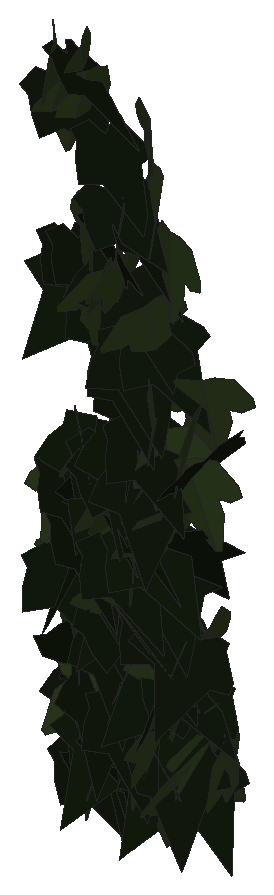
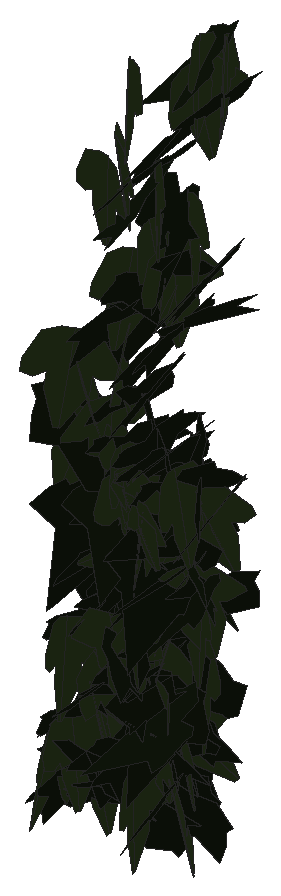
# SketchUp Ruby script. Lengths in inches.
U = 1.inch
M = Sketchup.active_model
def pt(a) = Geom::Point3d.new(a.map { |v| v * U })
def face(e, loops, mat)
  f = e.add_face(loops[0].map { |a| pt(a) })
  loops[1..].each { |l| e.add_face(l.map { |a| pt(a) }).erase! }
  f.material = f.back_material = mat if mat
  f
end
# faces: each face lists its corners as indices into pts; further lists are holes
def faces(e, pts, list, mat = nil) = list.each { |f| face(e, (f[0].is_a?(Array) ? f : [f]).map { |l| l.map { |i| pts[i] } }, mat) }
# xy, xz, yz: faces in a plane at the given z, y or x. An outline is a flat list of corners, or four numbers for a rectangle; further outlines are holes
def ring(l) = l.size == 4 ? [[l[0], l[1]], [l[2], l[1]], [l[2], l[3]], [l[0], l[3]]] : l.each_slice(2).to_a
def flat(e, list, mat, &to3) = list.each { |f| face(e, (f[0].is_a?(Array) ? f : [f]).map { |l| ring(l).map { |u, v| to3.(u, v) } }, mat) }
def xy(e, z, list, mat = nil) = flat(e, list, mat) { |x, y| [x, y, z] }
def xz(e, y, list, mat = nil) = flat(e, list, mat) { |x, z| [x, y, z] }
def yz(e, x, list, mat = nil) = flat(e, list, mat) { |y, z| [x, y, z] }
def lines(e, pts, list) = list.each { |a, b| e.add_line(pt(pts[a]), pt(pts[b])) }
# prism: a flat outline (further loops are holes) pulled along v
def prism(e, loops, v, mat = nil)
  f = face(e, loops, mat); d = Geom::Vector3d.new(v.map { |x| x * U })
  f.pushpull(f.normal.samedirection?(d) ? d.length : -d.length)
end
def box(e, o, s, mat = nil) = prism(e, [[o, [o[0] + s[0], o[1], o[2]], [o[0] + s[0], o[1] + s[1], o[2]], [o[0], o[1] + s[1], o[2]]]], [0, 0, s[2]], mat)
def at(x, y, z, deg = 0) = Geom::Transformation.translation(pt([x, y, z])) * Geom::Transformation.rotation(ORIGIN, Z_AXIS, deg.degrees)
def axes(o, x, y, z) = Geom::Transformation.new([*x, 0, *y, 0, *z, 0, *pt(o).to_a, 1])
def part(name) = M.definitions.add(name)
# library, detail: a bought-in or finely detailed component or shape, given as its bounding box
def library(name, o, s) = part(name).tap { |d| box(d.entities, o, s) }
def detail(e, o, s) = box(e.add_group.entities, o, s)
def put(e, d, t, mat = nil) = e.add_instance(d, t).tap { |i| i.material = mat if mat }
def group(e, t, mat = nil) = e.add_group.tap { |g| g.transformation = t; g.material = mat if mat }.entities
root = M.entities
M.materials.add("efeu1").color = [18, 25, 13]
M.materials.add("efeu2").color = [43, 57, 29]
c1 = part("ivyleaf_10")
p = [[0,0.5,-0.03],[-0.0625,2.02,-0.43],[-0.19,2.01,-0.46],[-0.54,1.05,-0.29],[-0.52,0.625,-0.18],[-0.83,0.76,-0.28],
  [-1.16,0.64,-0.33],[-1.15,0.33,-0.24],[-0.77,-0.39,0.02],[-0.3,-0.51,0.16],[0.04,-0.48,0.23],[-0.02,2.01,-0.4375],
  [-0.06,2.01,-0.43],[0.04,-0.49,0.23],[0.67,-0.49,0.14],[1.38,0.36,-0.2],[1.375,0.51,-0.24],[0.81,0.65,-0.19],
  [0.62,0.59,-0.15],[0.6,1.09,-0.28],[0.5,1.23,-0.31]]
faces(c1.entities,p,[[0,1,2,3,4,5,6,7,8,9,10],[11,12,0,13,14,15,16,17,18,19,20]],"efeu2")
c2 = part("ivyleaf_9")
p = [[1.54,2.16,1.25],[1.36,2.04,1.19],[-0.21,0.99,0.68],[-0.71,1.11,0.82],[-0.85,0.86,0.67],[-0.8,0.17,0.21],
  [-0.9,-0.01,0.1],[-0.67,-0.16,-0.02],[-0.08,-0.08,-0.05],[-0.03,-0.6,-0.4],[0.65,-0.88,-0.66],[0.83,-0.6,-0.49],
  [1.29,-0.42,-0.43],[1.8125,-0.07,-0.26],[1.21,0.44,0.15]]
faces(c2.entities,p,[[0,1,2,3,4,5,6,7,8,9,10,11,12,13,14]],"efeu1")
put(root,c1,axes([16.36,223.625,233.52],[0.23631,-0.40338,-0.17731],[0.01885,0.21027,-0.45324],[0.44023,0.20753,0.11459]))
put(root,c1,axes([16.68,224.23,224.14],[-0.34276,-0.05876,0.35925],[-0.26013,-0.30565,-0.29818],[0.25465,-0.39131,0.17896]))
put(root,c1,axes([16.51,223.875,224.82],[0.3091,-0.25368,-0.30017],[-0.09702,0.32081,-0.37103],[0.38084,0.28762,0.1491]))
put(root,c1,axes([16.57,224.01,225.79],[-0.41513,0.23915,0.1431],[-0.16261,0.00065,-0.47282],[-0.22633,-0.4391,0.07724]))
put(root,c1,axes([16.5,223.97,227.23],[0.42817,0.18988,-0.17497],[-0.17477,-0.03628,-0.46705],[-0.19007,0.46112,0.0353]))
put(root,c1,axes([16.59,224.15,226.13],[-0.37301,-0.2749,0.18786],[-0.09895,-0.17783,-0.45671],[0.31791,-0.3779,0.07826]))
put(root,c1,axes([16.54,224.35,227.62],[0.01144,-0.49941,-0.02146],[0.0006,0.02148,-0.49954],[0.49987,0.0114,0.0011]))
put(root,c1,axes([16.54,224.35,224.21],[0.31577,-0.36915,-0.1184],[-0.05573,0.1079,-0.48503],[0.38365,0.31951,0.027]))
put(root,c2,axes([16.54,224.18,229.95],[-0.30358,-0.34379,0.19911],[-0.01218,-0.24241,-0.43714],[0.3971,-0.27026,0.13881]))
put(root,c2,axes([16.3,223.8125,233.03],[0.23243,-0.37753,-0.23119],[-0.00634,0.25825,-0.4281],[0.44265,0.20194,0.11526]))
put(root,c2,axes([16.32,223.96,227.17],[0.2145,-0.44997,-0.03894],[-0.0152,0.03589,-0.49848],[0.45139,0.21504,0.00172]))
put(root,c2,axes([16.6,224.04,226.47],[-0.36619,0.11606,-0.32005],[0.28886,-0.14284,-0.3823],[-0.18017,-0.46489,0.03757]))
put(root,c2,axes([16.42,223.88,226.05],[-0.01712,-0.3956,-0.3053],[0.01443,0.30496,-0.39597],[0.4995,-0.02237,0.00097]))
put(root,c2,axes([16.35,224,230.5625],[0.21139,-0.4458,-0.0811],[-0.01887,0.08076,-0.49307],[0.45272,0.21153,0.01732]))
put(root,c2,axes([16.29,224.72,224.5625],[0.46602,-0.17972,-0.023],[0.04122,0.16698,-0.46949],[0.17644,0.43568,0.17044]))
put(root,c2,axes([16.45,223.98,226.22],[0.44251,-0.14345,-0.18333],[-0.1495,0.1267,-0.46],[0.17843,0.46192,0.06924]))
put(root,c1,axes([16.5625,224.32,224.05],[0.03575,0.4985,-0.01489],[-0.00064,-0.01489,-0.49978],[-0.49872,0.03575,-0.00042]))
put(root,c2,axes([16.62,224.4,224.64],[0.40758,0.24782,-0.14987],[-0.18534,0.02437,-0.46374],[-0.22254,0.43358,0.11173]))
put(root,c2,axes([16.39,224.16,230.51],[0.22114,-0.44173,-0.07729],[0.00508,0.08865,-0.49205],[0.44841,0.21684,0.0437]))
put(root,c2,axes([16.25,224.125,224.36],[0.16586,-0.02978,0.47075],[0.47156,-0.00133,-0.16623],[0.01115,0.49911,0.02765]))
put(root,c1,axes([16.66,223.76,233.48],[0.1131,-0.45719,-0.1679],[0.01562,0.17568,-0.46786],[0.48679,0.10059,0.05402]))
put(root,c1,axes([16.7,223.8,233.09],[-0.10581,-0.48456,0.06328],[0.00095,-0.06495,-0.49576],[0.48867,-0.1048,0.01467]))
put(root,c2,axes([16.9,223.6,227.79],[0.05176,0.11866,-0.48295],[-0.48804,0.10546,-0.0264],[0.0956,0.47413,0.12674]))
put(root,c2,axes([16.65,224.27,224.17],[-0.41082,-0.20004,-0.20299],[0.17385,0.1063,-0.45659],[0.22583,-0.44574,-0.01778]))
put(root,c1,axes([16.66,224.55,224.54],[-0.36664,0.32625,-0.09557],[-0.00494,-0.14566,-0.47829],[-0.33993,-0.34977,0.11004]))
put(root,c2,axes([16.72,224.68,224.11],[-0.45308,-0.10094,-0.18582],[0.19076,-0.00546,-0.46215],[0.09127,-0.48967,0.04346]))
put(root,c1,axes([16.69,224.21,223.12],[0.26545,-0.42232,-0.03439],[-0.01362,0.03206,-0.49879],[0.4235,0.26574,0.00551]))
put(root,c2,axes([16.66,224.29,227.63],[-0.23156,-0.43996,-0.05308],[0.01919,0.04988,-0.49714],[0.44273,-0.23227,-0.00622]))
put(root,c2,axes([16.46,224.125,223.17],[-0.10406,-0.11713,-0.47482],[0.42817,0.21276,-0.14632],[0.23632,-0.43705,0.05602]))
put(root,c2,axes([16.55,223.8125,226.56],[0.26733,-0.42153,-0.02914],[-0.01194,0.02693,-0.49913],[0.42236,0.26757,0.00433]))
put(root,c1,axes([16.85,223.71,231.17],[0.36155,-0.30354,-0.16475],[-0.03421,0.20587,-0.45437],[0.34367,0.33983,0.12809]))
put(root,c2,axes([16.6,223.71,227.03],[0.36098,0.21153,0.27376],[0.22527,0.15656,-0.41802],[-0.26257,0.42514,0.01772]))
put(root,c2,axes([16.54,223.77,233.44],[0.35383,-0.35318,-0.00832],[0.04805,0.05979,-0.49408],[0.34999,0.34884,0.07625]))
put(root,c2,axes([16.92,224.26,226.34],[0.16072,0.46754,0.07471],[-0.00133,0.07934,-0.49366],[-0.47346,0.15848,0.02675]))
put(root,c2,axes([16.7,224.19,223.97],[0.04203,-0.47931,0.13601],[0.00957,-0.13569,-0.48114],[0.49814,0.04305,-0.00224]))
put(root,c2,axes([16.97,224.26,223.52],[-0.33876,-0.36426,0.05057],[-0.03199,-0.03931,-0.49742],[0.36636,-0.34025,0.00333]))
put(root,c2,axes([16.72,224.65,223.12],[0.07794,-0.46272,0.17267],[0.01057,-0.1732,-0.46892],[0.49377,0.07675,-0.01722]))
put(root,c1,axes([16.88,224,225.65],[-0.15702,0.46815,0.0786],[-0.02222,0.07545,-0.49377],[-0.47418,-0.15856,-0.00289]))
put(root,c2,axes([16.72,224.18,229.75],[0.14632,-0.47478,-0.05631],[-0.00085,0.05863,-0.49655],[0.47811,0.14541,0.01635]))
put(root,c2,axes([17,223.96,223.64],[0.07546,-0.00557,0.49424],[0.06365,0.49592,-0.00413],[-0.49016,0.06354,0.07555]))
put(root,c1,axes([16.98,224.67,223.32],[0.07984,-0.47978,-0.11593],[0.02734,0.12156,-0.48423],[0.49283,0.07098,0.04564]))
put(root,c2,axes([16.74,224.44,226.26],[0.20193,-0.41741,-0.18707],[0.0333,0.21736,-0.44905],[0.45619,0.1689,0.11558]))
put(root,c1,axes([17.07,223.82,230.36],[-0.12169,-0.48463,-0.01811],[-0.00185,0.01914,-0.49963],[0.48496,-0.12154,-0.00645]))
put(root,c2,axes([16.875,224.63,223.85],[-0.03496,-0.4695,-0.16837],[0.02715,0.16674,-0.4706],[0.49804,-0.04204,0.01384]))
put(root,c2,axes([16.85,224.38,224.25],[-0.20643,-0.00794,-0.45533],[0.45363,-0.04761,-0.20483],[-0.0401,-0.49767,0.02686]))
put(root,c1,axes([17.09,224.04,227.18],[-0.11545,-0.46221,-0.15178],[0.03603,0.14744,-0.47641],[0.48515,-0.12094,-0.00073]))
put(root,c1,axes([17.22,223.46,230.13],[0.00313,0.07173,0.49482],[-0.28543,0.40653,-0.05713],[-0.41051,-0.28212,0.04349]))
put(root,c1,axes([17.1,224.54,225.33],[-0.14657,-0.42271,0.22323],[0.02581,-0.24014,-0.4378],[0.47734,-0.11681,0.09222]))
put(root,c1,axes([17.09,224.36,227.01],[0.20046,-0.41504,-0.19379],[0.03824,0.22596,-0.44439],[0.45646,0.16335,0.12234]))
put(root,c2,axes([16.71,224.06,222.73],[0.07402,-0.11321,0.48136],[0.4075,-0.26175,-0.12422],[0.28011,0.4107,0.05351]))
put(root,c1,axes([17.12,224.25,225.21],[0.0755,-0.48148,0.11172],[0.02739,-0.10876,-0.48726],[0.49351,0.0797,0.00995]))
put(root,c2,axes([16.79,224,227.16],[0.25257,-0.37364,0.21588],[0.11578,-0.18229,-0.45096],[0.4157,0.27778,-0.00556]))
put(root,c2,axes([16.9375,224.16,224.92],[0.05338,-0.49709,0.00751],[0.00076,-0.00748,-0.49994],[0.49714,0.05339,-0.00004]))
put(root,c1,axes([17.21,223.91,225.875],[-0.06233,-0.46353,0.17679],[-0.02741,-0.17469,-0.46769],[0.49534,-0.06799,-0.00364]))
put(root,c1,axes([16.875,224.22,225.17],[0.40367,-0.02499,0.29398],[0.29468,0.05877,-0.39964],[-0.01458,0.4959,0.06218]))
put(root,c2,axes([17.02,224.41,225.1],[-0.0856,-0.45213,-0.19557],[0.03669,0.1921,-0.46016],[0.49125,-0.09314,0.00029]))
put(root,c1,axes([17.33,224.38,227.3125],[0.38423,-0.10331,-0.30282],[-0.24985,0.19873,-0.38482],[0.19987,0.44703,0.10109]))
put(root,c2,axes([17.21,223.55,231.15],[0.37415,0.05108,-0.32772],[-0.33052,0.01625,-0.37482],[-0.02764,0.49712,0.04593]))
put(root,c2,axes([16.97,224.03,227.84],[0.11194,-0.42738,-0.23414],[0.02691,0.24529,-0.43487],[0.48656,0.08476,0.07792]))
put(root,c2,axes([16.97,223.98,232.3125],[0.19127,-0.44788,-0.11323],[-0.00208,0.12172,-0.48495],[0.46196,0.18599,0.0447]))
put(root,c2,axes([17.33,224.58,225.35],[-0.30979,0.26021,-0.29381],[0.23179,-0.18076,-0.40448],[-0.31671,-0.38681,-0.00863]))
put(root,c2,axes([17.36,224.17,225.98],[-0.43284,-0.2496,-0.01874],[0.01705,0.00796,-0.49965],[0.24972,-0.43317,0.00162]))
put(root,c2,axes([17.0625,223.7,225.62],[0.33978,-0.22976,-0.28593],[-0.10303,0.31428,-0.37498],[0.35204,0.31374,0.16623]))
put(root,c1,axes([17.25,224.39,227.13],[0.44902,-0.21785,-0.03043],[-0.02672,0.01463,-0.49907],[0.21833,0.44981,0.0015]))
put(root,c1,axes([17.32,223.86,230.66],[0.04343,-0.49733,-0.02792],[-0.0037,0.0277,-0.49922],[0.4981,0.04357,-0.00128]))
put(root,c1,axes([17.19,223.8125,226.82],[0.03705,-0.35712,0.34798],[0.019,0.3497,0.35686],[-0.49826,-0.01321,0.03948]))
put(root,c2,axes([17.22,224.125,230.34],[-0.17561,-0.46068,-0.08329],[0.01313,0.08408,-0.49271],[0.46796,-0.17524,-0.01743]))
put(root,c1,axes([17.39,224.17,227.29],[-0.32253,-0.37402,0.078],[-0.03017,-0.07682,-0.49314],[0.38087,-0.32282,0.02699]))
put(root,c2,axes([17.05,223.75,227.78],[0.29264,-0.33993,-0.22092],[-0.00448,0.26974,-0.42098],[0.40539,0.24837,0.15483]))
put(root,c1,axes([17.37,223.73,231.47],[0.25753,-0.348,-0.25015],[-0.06164,0.25873,-0.42339],[0.42412,0.24891,0.09035]))
put(root,c2,axes([17.16,224.17,228.72],[0.15718,-0.47444,0.01421],[0.00367,-0.01375,-0.4998],[0.47464,0.15723,-0.00084]))
put(root,c2,axes([17.25,223.95,228.0625],[-0.25886,0.02159,-0.42723],[0.42432,-0.0504,-0.25964],[-0.05427,-0.49698,0.00777]))
put(root,c1,axes([17.375,224.58,225.44],[0.49174,0.08138,-0.03958],[-0.05415,0.08938,-0.48896],[-0.07251,0.48517,0.09672]))
put(root,c2,axes([17.01,224.53,225.39],[0.34637,-0.03393,-0.359],[0.35745,0.0979,0.33562],[0.04752,-0.48915,0.09207]))
put(root,c1,axes([17.52,223.6875,226.67],[0.31014,-0.25067,-0.30162],[-0.13363,0.29399,-0.38173],[0.36872,0.31739,0.11536]))
put(root,c2,axes([17.27,224.56,223.84],[-0.05742,-0.44721,-0.21611],[0.0453,0.21192,-0.4506],[0.49462,-0.07133,0.01618]))
put(root,c2,axes([17.34,224.01,227.875],[-0.0498,-0.49615,0.03675],[-0.00236,-0.03669,-0.49865],[0.49751,-0.04984,0.00131]))
put(root,c2,axes([17.27,223.94,229.23],[0.14037,-0.4741,-0.07434],[-0.0067,0.07551,-0.49422],[0.47985,0.13974,0.01484]))
put(root,c2,axes([17.29,223.91,224.11],[0.09198,-0.48003,-0.10542],[-0.01899,0.1037,-0.48876],[0.4911,0.09391,0.00085]))
put(root,c2,axes([17.62,224.19,226.89],[0.07269,0.46319,0.17369],[-0.04977,0.18151,-0.46322],[-0.49218,0.05006,0.07249]))
put(root,c1,axes([17.24,224.2,225.86],[0.39097,-0.05488,0.30681],[0.31137,0.04679,-0.38841],[0.01392,0.49477,0.07076]))
put(root,c1,axes([17.32,223.9,226.45],[0.06577,-0.11216,-0.4828],[0.31399,0.38627,-0.04696],[0.38352,-0.29701,0.12125]))
put(root,c2,axes([17.29,223.67,231.76],[0.25217,-0.38127,-0.2026],[0.03396,0.25141,-0.43086],[0.43042,0.20354,0.15269]))
put(root,c2,axes([17.34,223.75,226.55],[0.11242,-0.44828,-0.1908],[0.02948,0.20171,-0.45655],[0.4863,0.0914,0.07178]))
put(root,c1,axes([17.66,224.46,224.74],[-0.10481,-0.43338,0.22626],[0.02203,-0.23535,-0.4406],[0.48839,-0.08239,0.06843]))
put(root,c2,axes([17.38,224.16,225.74],[0.02837,-0.37718,-0.327],[0.11933,0.32316,-0.3624],[0.48472,-0.05747,0.10836]))
put(root,c2,axes([17.65,224.55,223.18],[-0.29593,-0.39376,0.08587],[-0.02433,-0.08889,-0.49143],[0.40228,-0.29504,0.03346]))
put(root,c1,axes([17.66,224.02,227.41],[0.06952,-0.49117,-0.06262],[0.00326,0.06368,-0.49592],[0.49513,0.06855,0.01205]))
put(root,c2,axes([17.64,224.35,224.46],[-0.23496,-0.34005,0.28136],[-0.04636,-0.29796,-0.39884],[0.43891,-0.21351,0.10848]))
put(root,c2,axes([17.39,224.03,231.29],[0.27306,-0.41883,0.00445],[0.02463,0.01075,-0.49928],[0.41813,0.27289,0.02651]))
put(root,c1,axes([17.73,223.82,232.78],[0.32607,-0.32297,-0.19841],[-0.0125,0.25242,-0.43143],[0.37884,0.28631,0.15654]))
put(root,c2,axes([17.48,223.95,227.08],[0.29016,-0.399,-0.08129],[-0.03552,0.07463,-0.49312],[0.40564,0.29194,0.01496]))
put(root,c2,axes([17.97,224.82,223.54],[-0.49279,-0.04884,0.06909],[-0.06773,-0.01698,-0.4951],[0.05071,-0.49732,0.01012]))
put(root,c2,axes([17.45,223.83,225.5],[0.44787,-0.22229,0.00039],[0.00044,0.00002,-0.5],[0.22229,0.44787,0.00022]))
put(root,c1,axes([17.76,223.8,230.08],[-0.20647,-0.43129,-0.14615],[0.06265,0.13204,-0.47816],[0.45105,-0.21577,-0.00049]))
put(root,c2,axes([17.61,223.86,229.59],[-0.06323,-0.44681,-0.21531],[0.04189,0.21147,-0.45114],[0.49421,-0.07509,0.01069]))
put(root,c1,axes([17.76,223.99,231.81],[0.33294,-0.37186,-0.0296],[0.02819,0.06465,-0.495],[0.37197,0.32794,0.06401]))
put(root,c1,axes([17.77,223.97,223.9],[0.12296,-0.45287,0.1726],[0.05874,-0.16283,-0.46908],[0.48107,0.13563,0.01316]))
put(root,c2,axes([17.48,224.23,223.47],[0.12782,-0.24994,0.41375],[0.20189,-0.36125,-0.2806],[0.43921,0.2388,0.00857]))
put(root,c1,axes([17.96,223.65,228.69],[0.02988,-0.06737,-0.49454],[-0.13278,0.4765,-0.07293],[0.48112,0.13568,0.01058]))
put(root,c2,axes([17.59,224.54,224.57],[0.2215,-0.41092,-0.17911],[0.04885,0.22072,-0.44598],[0.44559,0.18007,0.13793]))
put(root,c2,axes([17.65,224.14,229.64],[0.12323,-0.41299,-0.25349],[0.01477,0.26463,-0.42397],[0.48435,0.09701,0.07743]))
put(root,c2,axes([17.77,223.89,227.71],[-0.14184,-0.46912,-0.09903],[0.03652,0.0924,-0.49003],[0.47807,-0.14624,0.00805]))
put(root,c2,axes([17.7,223.79,228.38],[0.1176,-0.43962,-0.20712],[-0.0222,0.20802,-0.45413],[0.48547,0.11601,0.02941]))
put(root,c1,axes([17.93,224.35,224.42],[0.26438,-0.42151,-0.04929],[-0.02024,0.04549,-0.49751],[0.4239,0.26506,0.00699]))
put(root,c1,axes([17.95,223.8125,227.1],[-0.14002,-0.47503,-0.06884],[0.01881,0.06622,-0.49524],[0.47962,-0.14128,-0.00067]))
put(root,c2,axes([17.76,224.28,226.27],[-0.02975,-0.47387,-0.15672],[0.01366,0.15617,-0.47479],[0.49893,-0.03253,0.00365]))
put(root,c2,axes([17.88,224.76,224.26],[-0.21179,-0.44415,0.08875],[-0.00973,-0.09349,-0.49109],[0.45282,-0.20974,0.03096]))
put(root,c2,axes([17.71,224.09,225.54],[0.11469,-0.45919,-0.16122],[0.00893,0.16759,-0.47099],[0.48659,0.10516,0.04664]))
put(root,c1,axes([17.97,224.65,223.82],[-0.11617,-0.48523,-0.03245],[0.00984,0.03101,-0.49894],[0.48622,-0.11656,0.00235]))
put(root,c2,axes([17.8,223.7,224.15],[-0.07301,0.42233,0.2575],[0.01568,-0.25818,0.4279],[0.49439,0.07056,0.02445]))
put(root,c2,axes([17.71,223.89,226.8],[0.05773,-0.41784,-0.26847],[0.09012,0.2746,-0.40801],[0.48841,-0.00128,0.10702]))
put(root,c1,axes([17.94,223.99,228.11],[0.15134,0.4757,-0.02831],[-0.06859,-0.00765,-0.49521],[-0.47158,0.15377,0.06294]))
put(root,c1,axes([18.03,224.15,223.21],[0.01293,-0.4998,0.00538],[-0.00049,-0.00539,-0.49997],[0.49983,0.01293,-0.00063]))
put(root,c1,axes([18.06,224.67,225.12],[0.00651,-0.46317,-0.18824],[0.00709,0.18832,-0.46313],[0.49991,0.00336,0.00902]))
put(root,c2,axes([18.01,224.04,226.72],[0.39219,0.30811,-0.03542],[-0.02759,-0.02222,-0.49874],[-0.30891,0.39316,-0.00042]))
put(root,c2,axes([17.98,224.1875,223.56],[-0.12697,-0.46159,-0.14427],[0.04867,0.1362,-0.47862],[0.48116,-0.13558,0.01035]))
put(root,c1,axes([18.11,224.5,223.45],[0.02428,-0.40514,0.29202],[0.12737,-0.27767,-0.39582],[0.48289,0.09361,0.08972]))
put(root,c1,axes([18.23,223.76,231.24],[-0.45608,0.20485,0.00532],[-0.05789,-0.11634,-0.48282],[-0.19657,-0.44102,0.12984]))
put(root,c2,axes([17.98,224.57,223.26],[0.07639,-0.46926,-0.15479],[0.02403,0.15997,-0.47311],[0.49355,0.06484,0.04699]))
put(root,c2,axes([18.21,224.23,225.27],[-0.19994,-0.4471,0.10065],[-0.00259,-0.1087,-0.48803],[0.45828,-0.19567,0.04115]))
put(root,c1,axes([18.24,224.11,228.55],[0.27972,-0.40516,0.08718],[0.05531,-0.06774,-0.49229],[0.41073,0.28505,0.00693]))
put(root,c2,axes([18.47,224.08,228.08],[-0.10441,0.47938,-0.09643],[-0.00687,-0.10003,-0.48984],[-0.48893,-0.10096,0.02747]))
put(root,c1,axes([18.33,224.28,228.96],[-0.4294,-0.25216,-0.04505],[0.03504,0.02928,-0.49791],[0.25375,-0.43076,-0.00748]))
put(root,c1,axes([18.32,224.68,223.45],[0.13209,-0.41935,-0.23811],[0.06474,0.26007,-0.42211],[0.47787,0.08068,0.123]))
put(root,c1,axes([18.27,224.12,227.78],[-0.47108,-0.05208,-0.15927],[0.16664,-0.09555,-0.46163],[0.01765,-0.48801,0.10739]))
